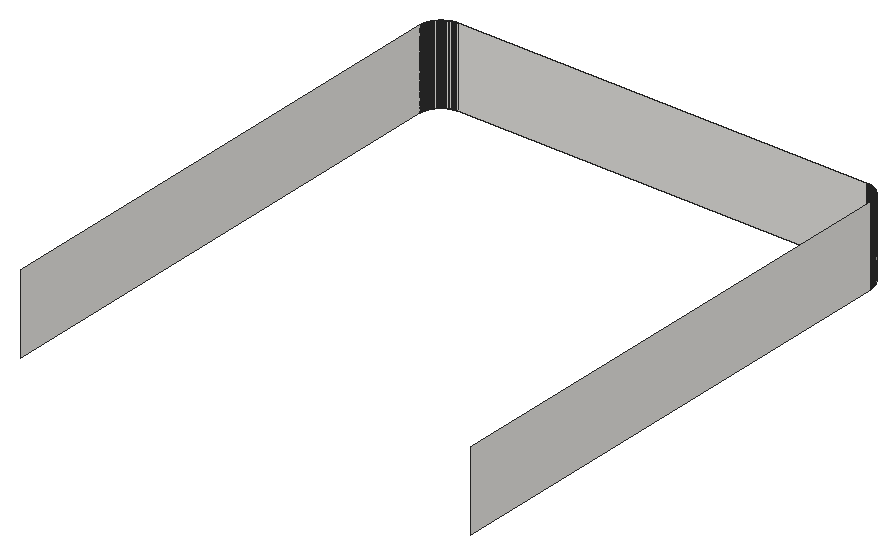
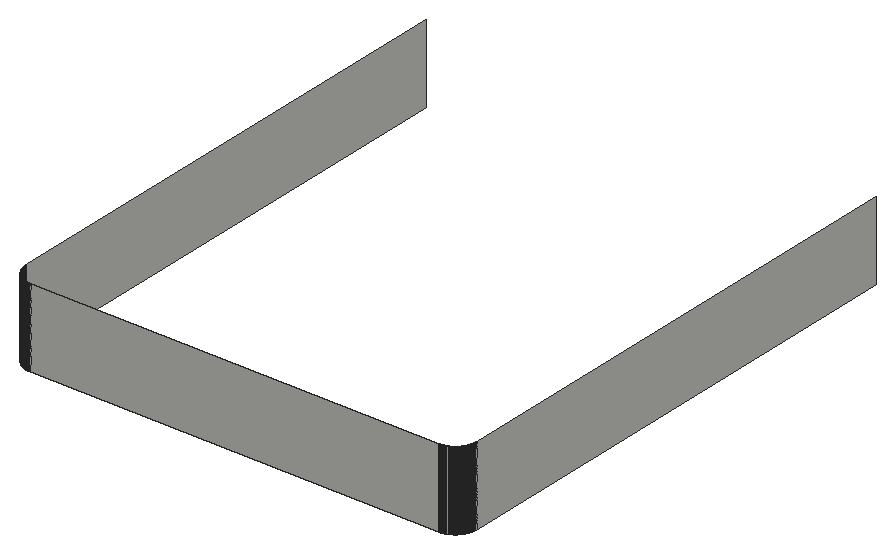
# SketchUp Ruby script. Lengths in inches.
U = 1.inch
M = Sketchup.active_model
def pt(a) = Geom::Point3d.new(a.map { |v| v * U })
def face(e, loops, mat)
  f = e.add_face(loops[0].map { |a| pt(a) })
  loops[1..].each { |l| e.add_face(l.map { |a| pt(a) }).erase! }
  f.material = f.back_material = mat if mat
  f
end
# faces: each face lists its corners as indices into pts; further lists are holes
def faces(e, pts, list, mat = nil) = list.each { |f| face(e, (f[0].is_a?(Array) ? f : [f]).map { |l| l.map { |i| pts[i] } }, mat) }
# xy, xz, yz: faces in a plane at the given z, y or x. An outline is a flat list of corners, or four numbers for a rectangle; further outlines are holes
def ring(l) = l.size == 4 ? [[l[0], l[1]], [l[2], l[1]], [l[2], l[3]], [l[0], l[3]]] : l.each_slice(2).to_a
def flat(e, list, mat, &to3) = list.each { |f| face(e, (f[0].is_a?(Array) ? f : [f]).map { |l| ring(l).map { |u, v| to3.(u, v) } }, mat) }
def xy(e, z, list, mat = nil) = flat(e, list, mat) { |x, y| [x, y, z] }
def xz(e, y, list, mat = nil) = flat(e, list, mat) { |x, z| [x, y, z] }
def yz(e, x, list, mat = nil) = flat(e, list, mat) { |y, z| [x, y, z] }
def lines(e, pts, list) = list.each { |a, b| e.add_line(pt(pts[a]), pt(pts[b])) }
# prism: a flat outline (further loops are holes) pulled along v
def prism(e, loops, v, mat = nil)
  f = face(e, loops, mat); d = Geom::Vector3d.new(v.map { |x| x * U })
  f.pushpull(f.normal.samedirection?(d) ? d.length : -d.length)
end
def box(e, o, s, mat = nil) = prism(e, [[o, [o[0] + s[0], o[1], o[2]], [o[0] + s[0], o[1] + s[1], o[2]], [o[0], o[1] + s[1], o[2]]]], [0, 0, s[2]], mat)
def at(x, y, z, deg = 0) = Geom::Transformation.translation(pt([x, y, z])) * Geom::Transformation.rotation(ORIGIN, Z_AXIS, deg.degrees)
def axes(o, x, y, z) = Geom::Transformation.new([*x, 0, *y, 0, *z, 0, *pt(o).to_a, 1])
def part(name) = M.definitions.add(name)
# library, detail: a bought-in or finely detailed component or shape, given as its bounding box
def library(name, o, s) = part(name).tap { |d| box(d.entities, o, s) }
def detail(e, o, s) = box(e.add_group.entities, o, s)
def put(e, d, t, mat = nil) = e.add_instance(d, t).tap { |i| i.material = mat if mat }
def group(e, t, mat = nil) = e.add_group.tap { |g| g.transformation = t; g.material = mat if mat }.entities
root = M.entities
M.materials.add("[Formica Graystone]").color = [224, 223, 219]
xz(root,439.98,[[17.37,392.82,17.48,422.82],[174.52,392.82,174.63,422.82]],"[Formica Graystone]")
xz(root,439.99,[[17.58,392.82,17.6875,422.82],[174.3125,392.82,174.42,422.82]],"[Formica Graystone]")
xz(root,440,[[17.79,392.82,17.9,422.82],[17.9,392.82,18,422.82],[18,392.82,174,422.82],[174,392.82,174.1,422.82],[174.1,392.82,174.21,422.82]],"[Formica Graystone]")
yz(root,10,[[241,392.82,432,422.82],[432,392.82,432.1,422.82],[432.1,392.82,432.21,422.82]],"[Formica Graystone]")
yz(root,10.01,[[432.3125,392.82,432.42,422.82]],"[Formica Graystone]")
yz(root,10.02,[[432.52,392.82,432.63,422.82]],"[Formica Graystone]")
yz(root,181.98,[[432.52,392.82,432.63,422.82]],"[Formica Graystone]")
yz(root,181.99,[[432.3125,392.82,432.42,422.82]],"[Formica Graystone]")
yz(root,182,[[241,392.82,432,422.82],[432,392.82,432.1,422.82],[432.1,392.82,432.21,422.82]],"[Formica Graystone]")
p = [[10.01,432.3125,392.82],[10,432.21,392.82],[10,432.21,422.82],[10.01,432.3125,422.82],[182,432.21,392.82],[181.99,432.3125,392.82],
  [181.99,432.3125,422.82],[182,432.21,422.82],[10.02,432.52,392.82],[10.01,432.42,392.82],[10.01,432.42,422.82],[10.02,432.52,422.82],
  [181.99,432.42,392.82],[181.98,432.52,392.82],[181.98,432.52,422.82],[181.99,432.42,422.82],[10.03,432.73,392.82],[10.02,432.63,392.82],
  [10.02,432.63,422.82],[10.03,432.73,422.82],[181.98,432.63,392.82],[181.97,432.73,392.82],[181.97,432.73,422.82],[181.98,432.63,422.82],
  [10.04,432.84,392.82],[10.04,432.84,422.82],[181.96,432.84,392.82],[181.96,432.84,422.82],[10.06,432.94,392.82],[10.06,432.94,422.82],
  [181.94,432.94,392.82],[181.94,432.94,422.82],[10.07,433.04,392.82],[10.07,433.04,422.82],[181.93,433.04,392.82],[181.93,433.04,422.82],
  [10.08,433.15,392.82],[10.08,433.15,422.82],[181.92,433.15,392.82],[181.92,433.15,422.82],[10.1,433.25,392.82],[10.1,433.25,422.82],
  [181.9,433.25,392.82],[181.9,433.25,422.82],[10.12,433.35,392.82],[10.12,433.35,422.82],[181.88,433.35,392.82],[181.88,433.35,422.82],
  [10.13,433.46,392.82],[10.13,433.46,422.82],[181.87,433.46,392.82],[181.87,433.46,422.82],[10.15,433.5625,392.82],[10.15,433.5625,422.82],
  [181.85,433.5625,392.82],[181.85,433.5625,422.82],[10.17,433.66,392.82],[10.17,433.66,422.82],[181.83,433.66,392.82],[181.83,433.66,422.82],
  [10.2,433.77,392.82],[10.2,433.77,422.82],[181.8,433.77,392.82],[181.8,433.77,422.82],[10.22,433.87,392.82],[10.22,433.87,422.82],
  [181.78,433.87,392.82],[181.78,433.87,422.82],[10.25,433.97,392.82],[10.25,433.97,422.82],[181.75,433.97,392.82],[181.75,433.97,422.82],
  [10.27,434.07,392.82],[10.27,434.07,422.82],[181.73,434.07,392.82],[181.73,434.07,422.82],[10.3,434.17,392.82],[10.3,434.17,422.82],
  [181.7,434.17,392.82],[181.7,434.17,422.82],[10.33,434.27,392.82],[10.33,434.27,422.82],[181.67,434.27,392.82],[181.67,434.27,422.82],
  [10.36,434.37,392.82],[10.36,434.37,422.82],[181.64,434.37,392.82],[181.64,434.37,422.82],[10.39,434.47,392.82],[10.39,434.47,422.82],
  [181.61,434.47,392.82],[181.61,434.47,422.82],[10.42,434.57,392.82],[10.42,434.57,422.82],[181.58,434.57,392.82],[181.58,434.57,422.82],
  [10.46,434.67,392.82],[10.46,434.67,422.82],[181.54,434.67,392.82],[181.54,434.67,422.82],[10.49,434.77,392.82],[10.49,434.77,422.82],
  [181.51,434.77,392.82],[181.51,434.77,422.82],[10.53,434.87,392.82],[10.53,434.87,422.82],[181.47,434.87,392.82],[181.47,434.87,422.82],
  [10.57,434.96,392.82],[10.57,434.96,422.82],[181.43,434.96,392.82],[181.43,434.96,422.82],[10.61,435.0625,392.82],[10.61,435.0625,422.82],
  [181.39,435.0625,392.82],[181.39,435.0625,422.82],[10.65,435.16,392.82],[10.65,435.16,422.82],[181.35,435.16,392.82],[181.35,435.16,422.82],
  [10.69,435.25,392.82],[10.69,435.25,422.82],[181.31,435.25,392.82],[181.31,435.25,422.82],[10.73,435.35,392.82],[10.73,435.35,422.82],
  [10.78,435.44,392.82],[10.78,435.44,422.82],[181.27,435.35,392.82],[181.22,435.44,392.82],[181.22,435.44,422.82],[181.27,435.35,422.82],
  [10.83,435.54,392.82],[10.83,435.54,422.82],[181.17,435.54,392.82],[181.17,435.54,422.82],[10.87,435.63,392.82],[10.87,435.63,422.82],
  [181.13,435.63,392.82],[181.13,435.63,422.82],[10.92,435.72,392.82],[10.92,435.72,422.82],[181.08,435.72,392.82],[181.08,435.72,422.82],
  [10.97,435.82,392.82],[10.97,435.82,422.82],[181.03,435.82,392.82],[181.03,435.82,422.82],[11.02,435.91,392.82],[11.02,435.91,422.82],
  [180.98,435.91,392.82],[180.98,435.91,422.82],[11.07,436,392.82],[11.07,436,422.82],[180.93,436,392.82],[180.93,436,422.82],
  [11.125,436.09,392.82],[11.125,436.09,422.82],[180.875,436.09,392.82],[180.875,436.09,422.82],[11.18,436.18,392.82],[11.18,436.18,422.82],
  [180.82,436.18,392.82],[180.82,436.18,422.82],[11.23,436.27,392.82],[11.23,436.27,422.82],[180.77,436.27,392.82],[180.77,436.27,422.82],
  [11.29,436.36,392.82],[11.29,436.36,422.82],[180.71,436.36,392.82],[180.71,436.36,422.82],[11.35,436.44,392.82],[11.35,436.44,422.82],
  [11.41,436.53,392.82],[11.41,436.53,422.82],[180.65,436.44,392.82],[180.59,436.53,392.82],[180.59,436.53,422.82],[180.65,436.44,422.82],
  [11.47,436.62,392.82],[11.47,436.62,422.82],[180.53,436.62,392.82],[180.53,436.62,422.82],[11.53,436.7,392.82],[11.53,436.7,422.82],
  [180.47,436.7,392.82],[180.47,436.7,422.82],[11.59,436.79,392.82],[11.59,436.79,422.82],[180.41,436.79,392.82],[180.41,436.79,422.82],
  [11.65,436.87,392.82],[11.65,436.87,422.82],[180.35,436.87,392.82],[180.35,436.87,422.82],[11.72,436.95,392.82],[11.72,436.95,422.82],
  [180.28,436.95,392.82],[180.28,436.95,422.82],[11.78,437.03,392.82],[11.78,437.03,422.82],[11.85,437.12,392.82],[11.85,437.12,422.82],
  [180.22,437.03,392.82],[180.22,437.03,422.82],[180.15,437.12,392.82],[180.15,437.12,422.82],[11.92,437.2,392.82],[11.92,437.2,422.82],
  [180.08,437.2,392.82],[180.08,437.2,422.82],[11.99,437.27,392.82],[11.99,437.27,422.82],[180.01,437.27,392.82],[180.01,437.27,422.82],
  [12.05,437.35,392.82],[12.05,437.35,422.82],[179.95,437.35,392.82],[179.95,437.35,422.82],[12.125,437.43,392.82],[12.125,437.43,422.82],
  [12.2,437.51,392.82],[12.2,437.51,422.82],[179.875,437.43,392.82],[179.8,437.51,392.82],[179.8,437.51,422.82],[179.875,437.43,422.82],
  [12.27,437.58,392.82],[12.27,437.58,422.82],[179.73,437.58,392.82],[179.73,437.58,422.82],[12.34,437.66,392.82],[12.34,437.66,422.82],
  [179.66,437.66,392.82],[179.66,437.66,422.82],[12.42,437.73,392.82],[12.42,437.73,422.82],[12.49,437.8,392.82],[12.49,437.8,422.82],
  [179.58,437.73,392.82],[179.51,437.8,392.82],[179.51,437.8,422.82],[179.58,437.73,422.82],[12.57,437.875,392.82],[12.57,437.875,422.82],
  [179.43,437.875,392.82],[179.43,437.875,422.82],[12.65,437.95,392.82],[12.65,437.95,422.82],[12.73,438.01,392.82],[12.73,438.01,422.82],
  [179.35,437.95,392.82],[179.27,438.01,392.82],[179.27,438.01,422.82],[179.35,437.95,422.82],[12.8,438.08,392.82],[12.8,438.08,422.82],
  [179.2,438.08,392.82],[179.2,438.08,422.82],[12.88,438.15,392.82],[12.88,438.15,422.82],[179.12,438.15,392.82],[179.12,438.15,422.82],
  [12.97,438.22,392.82],[12.97,438.22,422.82],[13.05,438.28,392.82],[13.05,438.28,422.82],[179.03,438.22,392.82],[179.03,438.22,422.82],
  [178.95,438.28,392.82],[178.95,438.28,422.82],[13.13,438.35,392.82],[13.13,438.35,422.82],[13.21,438.41,392.82],[13.21,438.41,422.82],
  [178.87,438.35,392.82],[178.79,438.41,392.82],[178.79,438.41,422.82],[178.87,438.35,422.82],[13.3,438.47,392.82],[13.3,438.47,422.82],
  [178.7,438.47,392.82],[178.7,438.47,422.82],[13.38,438.53,392.82],[13.38,438.53,422.82],[13.47,438.59,392.82],[13.47,438.59,422.82],
  [178.62,438.53,392.82],[178.53,438.59,392.82],[178.53,438.59,422.82],[178.62,438.53,422.82],[13.56,438.65,392.82],[13.56,438.65,422.82],
  [178.44,438.65,392.82],[178.44,438.65,422.82],[13.64,438.71,392.82],[13.64,438.71,422.82],[13.73,438.77,392.82],[13.73,438.77,422.82],
  [178.36,438.71,392.82],[178.27,438.77,392.82],[178.27,438.77,422.82],[178.36,438.71,422.82],[13.82,438.82,392.82],[13.82,438.82,422.82],
  [13.91,438.875,392.82],[13.91,438.875,422.82],[178.18,438.82,392.82],[178.09,438.875,392.82],[178.09,438.875,422.82],[178.18,438.82,422.82],
  [14,438.93,392.82],[14,438.93,422.82],[14.09,438.98,392.82],[14.09,438.98,422.82],[178,438.93,392.82],[177.91,438.98,392.82],
  [177.91,438.98,422.82],[178,438.93,422.82],[14.18,439.03,392.82],[14.18,439.03,422.82],[14.28,439.08,392.82],[14.28,439.08,422.82],
  [177.82,439.03,392.82],[177.72,439.08,392.82],[177.72,439.08,422.82],[177.82,439.03,422.82],[14.37,439.13,392.82],[14.37,439.13,422.82],
  [14.46,439.17,392.82],[14.46,439.17,422.82],[177.63,439.13,392.82],[177.54,439.17,392.82],[177.54,439.17,422.82],[177.63,439.13,422.82],
  [14.56,439.22,392.82],[14.56,439.22,422.82],[14.65,439.27,392.82],[14.65,439.27,422.82],[177.44,439.22,392.82],[177.35,439.27,392.82],
  [177.35,439.27,422.82],[177.44,439.22,422.82],[14.75,439.31,392.82],[14.75,439.31,422.82],[14.84,439.35,392.82],[14.84,439.35,422.82],
  [177.25,439.31,392.82],[177.16,439.35,392.82],[177.16,439.35,422.82],[177.25,439.31,422.82],[14.9375,439.39,392.82],[14.9375,439.39,422.82],
  [15.04,439.43,392.82],[15.04,439.43,422.82],[15.13,439.47,392.82],[15.13,439.47,422.82],[176.96,439.43,392.82],[176.87,439.47,392.82],
  [176.87,439.47,422.82],[176.96,439.43,422.82],[177.0625,439.39,392.82],[177.0625,439.39,422.82],[15.23,439.51,392.82],[15.23,439.51,422.82],
  [15.33,439.54,392.82],[15.33,439.54,422.82],[15.43,439.58,392.82],[15.43,439.58,422.82],[176.67,439.54,392.82],[176.57,439.58,392.82],
  [176.57,439.58,422.82],[176.67,439.54,422.82],[176.77,439.51,392.82],[176.77,439.51,422.82],[15.53,439.61,392.82],[15.53,439.61,422.82],
  [15.63,439.64,392.82],[15.63,439.64,422.82],[15.73,439.67,392.82],[15.73,439.67,422.82],[176.37,439.64,392.82],[176.27,439.67,392.82],
  [176.27,439.67,422.82],[176.37,439.64,422.82],[176.47,439.61,392.82],[176.47,439.61,422.82],[15.83,439.7,392.82],[15.83,439.7,422.82],
  [15.93,439.73,392.82],[15.93,439.73,422.82],[16.03,439.75,392.82],[16.03,439.75,422.82],[176.07,439.73,392.82],[175.97,439.75,392.82],
  [175.97,439.75,422.82],[176.07,439.73,422.82],[176.17,439.7,392.82],[176.17,439.7,422.82],[16.13,439.78,392.82],[16.13,439.78,422.82],
  [16.23,439.8,392.82],[16.23,439.8,422.82],[16.34,439.83,392.82],[16.34,439.83,422.82],[16.4375,439.85,392.82],[16.4375,439.85,422.82],
  [16.54,439.87,392.82],[16.54,439.87,422.82],[175.5625,439.85,392.82],[175.46,439.87,392.82],[175.46,439.87,422.82],[175.5625,439.85,422.82],
  [175.66,439.83,392.82],[175.66,439.83,422.82],[175.77,439.8,392.82],[175.77,439.8,422.82],[175.87,439.78,392.82],[175.87,439.78,422.82],
  [16.65,439.88,392.82],[16.65,439.88,422.82],[16.75,439.9,392.82],[16.75,439.9,422.82],[16.85,439.92,392.82],[16.85,439.92,422.82],
  [16.96,439.93,392.82],[16.96,439.93,422.82],[17.06,439.94,392.82],[17.06,439.94,422.82],[17.16,439.96,392.82],[17.16,439.96,422.82],
  [174.94,439.94,392.82],[174.84,439.96,392.82],[174.84,439.96,422.82],[174.94,439.94,422.82],[175.04,439.93,392.82],[175.04,439.93,422.82],
  [175.15,439.92,392.82],[175.15,439.92,422.82],[175.25,439.9,392.82],[175.25,439.9,422.82],[175.35,439.88,392.82],[175.35,439.88,422.82],
  [17.27,439.97,392.82],[17.27,439.97,422.82],[17.37,439.98,392.82],[17.37,439.98,422.82],[17.58,439.99,392.82],[17.48,439.98,392.82],
  [17.48,439.98,422.82],[17.58,439.99,422.82],[17.79,440,392.82],[17.6875,439.99,392.82],[17.6875,439.99,422.82],[17.79,440,422.82],
  [174.3125,439.99,392.82],[174.21,440,392.82],[174.21,440,422.82],[174.3125,439.99,422.82],[174.52,439.98,392.82],[174.42,439.99,392.82],
  [174.42,439.99,422.82],[174.52,439.98,422.82],[174.73,439.97,392.82],[174.63,439.98,392.82],[174.63,439.98,422.82],[174.73,439.97,422.82]]
faces(root,p,[[0,1,2,3],[4,5,6,7],[8,9,10,11],[12,13,14,15],[16,17,18,19],[20,21,22,23],[24,16,19,25],[21,26,27,22],
  [28,24,25,29],[26,30,31,27],[32,28,29,33],[30,34,35,31],[36,32,33,37],[34,38,39,35],[40,36,37,41],[38,42,43,39],
  [44,40,41,45],[42,46,47,43],[48,44,45,49],[46,50,51,47],[52,48,49,53],[50,54,55,51],[56,52,53,57],[54,58,59,55],
  [60,56,57,61],[58,62,63,59],[64,60,61,65],[62,66,67,63],[68,64,65,69],[66,70,71,67],[72,68,69,73],[70,74,75,71],
  [76,72,73,77],[74,78,79,75],[80,76,77,81],[78,82,83,79],[84,80,81,85],[82,86,87,83],[88,84,85,89],[86,90,91,87],
  [92,88,89,93],[90,94,95,91],[96,92,93,97],[94,98,99,95],[100,96,97,101],[98,102,103,99],[104,100,101,105],[102,106,107,103],
  [108,104,105,109],[106,110,111,107],[112,108,109,113],[110,114,115,111],[116,112,113,117],[114,118,119,115],[120,116,117,121],[118,122,123,119],
  [124,120,121,125],[126,124,125,127],[128,129,130,131],[122,128,131,123],[132,126,127,133],[129,134,135,130],[136,132,133,137],[134,138,139,135],
  [140,136,137,141],[138,142,143,139],[144,140,141,145],[142,146,147,143],[148,144,145,149],[146,150,151,147],[152,148,149,153],[150,154,155,151],
  [156,152,153,157],[154,158,159,155],[160,156,157,161],[158,162,163,159],[164,160,161,165],[162,166,167,163],[168,164,165,169],[166,170,171,167],
  [172,168,169,173],[174,172,173,175],[176,177,178,179],[170,176,179,171],[180,174,175,181],[177,182,183,178],[184,180,181,185],[182,186,187,183],
  [188,184,185,189],[186,190,191,187],[192,188,189,193],[190,194,195,191],[196,192,193,197],[194,198,199,195],[200,196,197,201],[202,200,201,203],
  [198,204,205,199],[204,206,207,205],[208,202,203,209],[206,210,211,207],[212,208,209,213],[210,214,215,211],[216,212,213,217],[214,218,219,215],
  [220,216,217,221],[222,220,221,223],[224,225,226,227],[218,224,227,219],[228,222,223,229],[225,230,231,226],[232,228,229,233],[230,234,235,231],
  [236,232,233,237],[238,236,237,239],[240,241,242,243],[234,240,243,235],[244,238,239,245],[241,246,247,242],[248,244,245,249],[250,248,249,251],
  [252,253,254,255],[246,252,255,247],[256,250,251,257],[253,258,259,254],[260,256,257,261],[258,262,263,259],[264,260,261,265],[266,264,265,267],
  [262,268,269,263],[268,270,271,269],[272,266,267,273],[274,272,273,275],[276,277,278,279],[270,276,279,271],[280,274,275,281],[277,282,283,278],
  [284,280,281,285],[286,284,285,287],[288,289,290,291],[282,288,291,283],[292,286,287,293],[289,294,295,290],[296,292,293,297],[298,296,297,299],
  [300,301,302,303],[294,300,303,295],[304,298,299,305],[306,304,305,307],[308,309,310,311],[301,308,311,302],[312,306,307,313],[314,312,313,315],
  [316,317,318,319],[309,316,319,310],[320,314,315,321],[322,320,321,323],[324,325,326,327],[317,324,327,318],[328,322,323,329],[330,328,329,331],
  [332,333,334,335],[325,332,335,326],[336,330,331,337],[338,336,337,339],[340,341,342,343],[333,340,343,334],[344,338,339,345],[346,344,345,347],
  [348,349,350,351],[341,348,351,342],[352,346,347,353],[354,352,353,355],[356,354,355,357],[358,359,360,361],[362,358,361,363],[349,362,363,350],
  [364,356,357,365],[366,364,365,367],[368,366,367,369],[370,371,372,373],[374,370,373,375],[359,374,375,360],[376,368,369,377],[378,376,377,379],
  [380,378,379,381],[382,383,384,385],[386,382,385,387],[371,386,387,372],[388,380,381,389],[390,388,389,391],[392,390,391,393],[394,395,396,397],
  [398,394,397,399],[383,398,399,384],[400,392,393,401],[402,400,401,403],[404,402,403,405],[406,404,405,407],[408,406,407,409],[410,411,412,413],
  [414,410,413,415],[416,414,415,417],[418,416,417,419],[395,418,419,396],[420,408,409,421],[422,420,421,423],[424,422,423,425],[426,424,425,427],
  [428,426,427,429],[430,428,429,431],[432,433,434,435],[436,432,435,437],[438,436,437,439],[440,438,439,441],[442,440,441,443],[411,442,443,412],
  [444,430,431,445],[446,444,445,447],[448,449,450,451],[452,453,454,455],[456,457,458,459],[460,461,462,463],[464,465,466,467],[433,464,467,434]],"[Formica Graystone]")
